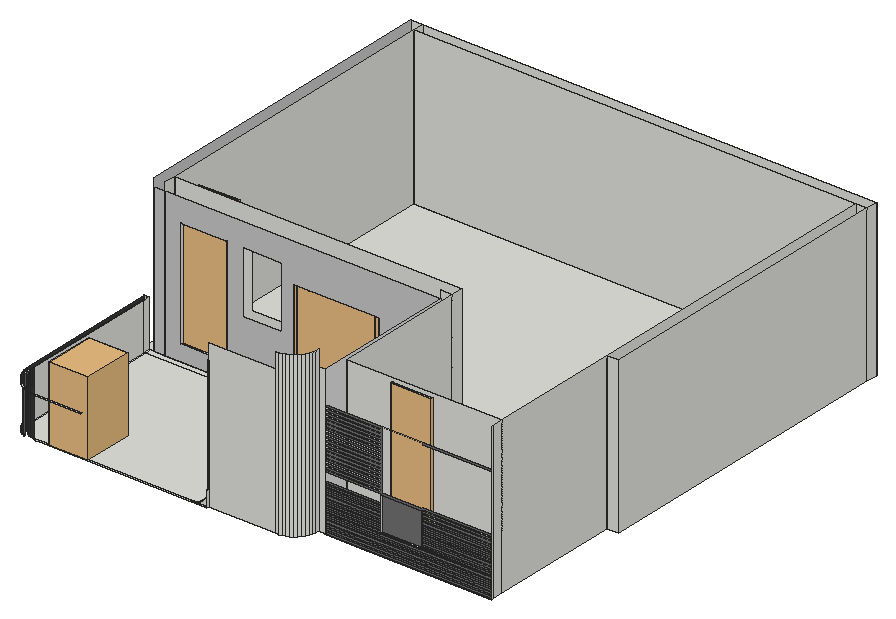
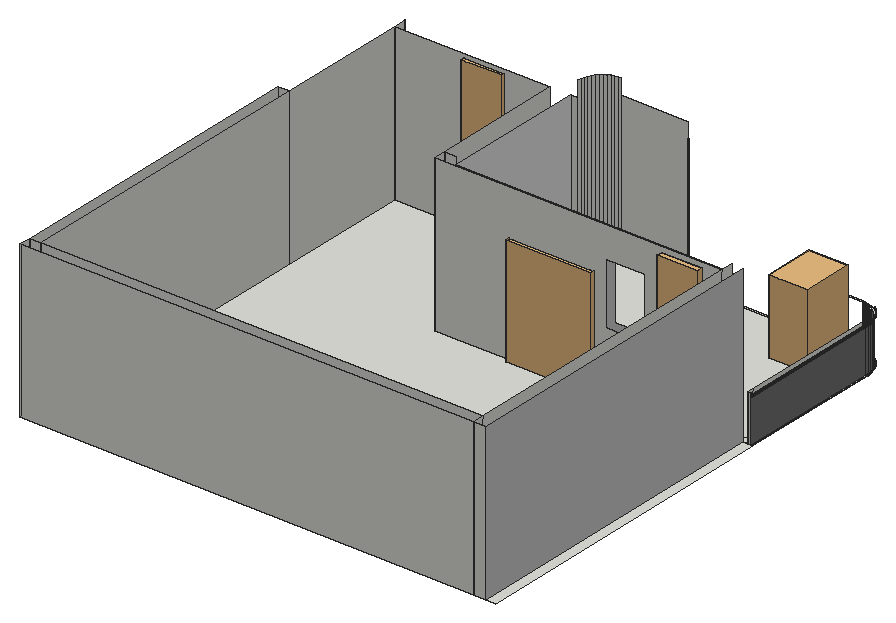
# SketchUp Ruby script. Lengths in inches.
U = 1.inch
M = Sketchup.active_model
def pt(a) = Geom::Point3d.new(a.map { |v| v * U })
def face(e, loops, mat)
  f = e.add_face(loops[0].map { |a| pt(a) })
  loops[1..].each { |l| e.add_face(l.map { |a| pt(a) }).erase! }
  f.material = f.back_material = mat if mat
  f
end
# faces: each face lists its corners as indices into pts; further lists are holes
def faces(e, pts, list, mat = nil) = list.each { |f| face(e, (f[0].is_a?(Array) ? f : [f]).map { |l| l.map { |i| pts[i] } }, mat) }
# xy, xz, yz: faces in a plane at the given z, y or x. An outline is a flat list of corners, or four numbers for a rectangle; further outlines are holes
def ring(l) = l.size == 4 ? [[l[0], l[1]], [l[2], l[1]], [l[2], l[3]], [l[0], l[3]]] : l.each_slice(2).to_a
def flat(e, list, mat, &to3) = list.each { |f| face(e, (f[0].is_a?(Array) ? f : [f]).map { |l| ring(l).map { |u, v| to3.(u, v) } }, mat) }
def xy(e, z, list, mat = nil) = flat(e, list, mat) { |x, y| [x, y, z] }
def xz(e, y, list, mat = nil) = flat(e, list, mat) { |x, z| [x, y, z] }
def yz(e, x, list, mat = nil) = flat(e, list, mat) { |y, z| [x, y, z] }
def lines(e, pts, list) = list.each { |a, b| e.add_line(pt(pts[a]), pt(pts[b])) }
# prism: a flat outline (further loops are holes) pulled along v
def prism(e, loops, v, mat = nil)
  f = face(e, loops, mat); d = Geom::Vector3d.new(v.map { |x| x * U })
  f.pushpull(f.normal.samedirection?(d) ? d.length : -d.length)
end
def box(e, o, s, mat = nil) = prism(e, [[o, [o[0] + s[0], o[1], o[2]], [o[0] + s[0], o[1] + s[1], o[2]], [o[0], o[1] + s[1], o[2]]]], [0, 0, s[2]], mat)
def at(x, y, z, deg = 0) = Geom::Transformation.translation(pt([x, y, z])) * Geom::Transformation.rotation(ORIGIN, Z_AXIS, deg.degrees)
def axes(o, x, y, z) = Geom::Transformation.new([*x, 0, *y, 0, *z, 0, *pt(o).to_a, 1])
def part(name) = M.definitions.add(name)
# library, detail: a bought-in or finely detailed component or shape, given as its bounding box
def library(name, o, s) = part(name).tap { |d| box(d.entities, o, s) }
def detail(e, o, s) = box(e.add_group.entities, o, s)
def put(e, d, t, mat = nil) = e.add_instance(d, t).tap { |i| i.material = mat if mat }
def group(e, t, mat = nil) = e.add_group.tap { |g| g.transformation = t; g.material = mat if mat }.entities
root = M.entities
M.materials.add("[Cladding Stucco White]").color = [200, 200, 200]
M.materials.add("[Color M01]").color = [226, 226, 226]
M.materials.add("[Color M05]").color = [114, 114, 114]
M.materials.add("[Color M07]").color = [58, 58, 58]
c1 = library("Potted Plant 02",[-16.98,-19.78,0],[30.04,38.68,37.52])
c2 = library("Curtains 004",[-15.59,-2.26,0],[31.18,4.52,116.91])
c3 = library("glass door",[0,-2.95,0],[39.37,5.9,82.68])
c4 = library("Door 243 053",[-21.6,-2.79,-0.07],[43.2,5.58,82.64])
xy(root,126,[[24.25,5.061,142.019,5.061,142.019,6.391,24.25,6.391,21.821,6.55,19.434,7.025,17.129,7.808,14.946,8.884,12.922,10.237,11.092,11.842,9.487,13.672,8.134,15.696,7.058,17.879,6.275,20.184,5.8,22.571,5.641,25,5.641,136,4.311,136,4.311,25,4.481,22.397,4.99,19.839,5.829,17.37,6.982,15.03,8.431,12.862,10.151,10.901,12.112,9.181,14.28,7.732,16.62,6.579,19.089,5.74,21.647,5.231],[142.019,5.061,154.019,6.391],[24.25,6.391,205.875,6.391,208.304,6.55,210.691,7.025,212.996,7.808,215.179,8.884,217.203,10.237,219.033,11.842,220.638,13.672,221.991,15.696,223.067,17.879,223.85,20.184,224.325,22.571,224.484,25,224.484,130.609,173.484,130.609,173.484,139.609,124.266,139.609,124.266,130.609,5.641,130.609,5.641,25,5.8,22.571,6.275,20.184,7.058,17.879,8.134,15.696,9.487,13.672,11.092,11.842,12.922,10.237,14.946,8.884,17.129,7.808,19.434,7.025,21.821,6.55],[229.875,24,238.875,25],[238.875,24,358.875,25],
  [224.484,25,229.875,25,229.875,136,178.875,136,178.875,145,118.875,145,118.875,136,5.641,136,5.641,130.609,124.266,130.609,124.266,139.609,173.484,139.609,173.484,130.609,224.484,130.609],[229.875,25,238.875,136],[238.875,25,358.875,34],[238.875,34,358.875,34,358.875,376,16.875,376,16.875,145,238.875,145],[0.25,136,7.875,385],
  [7.875,136,16.875,385],[16.875,136,118.875,145],[178.875,136,238.875,145],[358.875,136,367.875,376],[16.875,376,367.875,385]])
xy(root,126.103,[[12.811,5.186,12.812,5.189,10.324,6.851,10.322,6.849],[9.765,6.123,9.767,6.126,7.428,8.178,7.426,8.176],[10.322,6.849,10.324,6.851,8.074,8.824,8.072,8.822],[7.426,8.176,7.428,8.178,5.376,10.517,5.373,10.515],[8.072,8.822,8.074,8.824,6.101,11.074,6.099,11.072],
  [5.373,10.515,5.376,10.517,3.647,13.105,3.644,13.103],[6.099,11.072,6.101,11.074,4.439,13.562,4.436,13.561],[3.644,13.103,3.647,13.105,2.27,15.896,2.268,15.895],[4.436,13.561,4.439,13.562,3.115,16.246,3.113,16.245],[2.268,15.895,2.27,15.896,1.27,18.843,1.267,18.842],
  [3.113,16.245,3.115,16.246,2.153,19.079,2.151,19.078],[1.267,18.842,1.27,18.843,0.663,21.895,0.66,21.894],[2.151,19.078,2.153,19.079,1.57,22.014,1.567,22.014],[0.66,21.894,0.663,21.895,0.462,24.963,0.459,24.963],[0.459,24.963,0.462,24.963,0.459,25.007]])
xy(root,126.14,[[12.755,5.09,12.756,5.093,10.256,6.763,10.255,6.761],[9.833,6.211,9.835,6.214,7.506,8.256,7.504,8.254],[10.255,6.761,10.256,6.763,7.996,8.746,7.994,8.744],[7.504,8.254,7.506,8.256,5.464,10.585,5.461,10.583],[7.994,8.744,7.996,8.746,6.013,11.006,6.011,11.005],
  [5.461,10.583,5.464,10.585,3.743,13.16,3.74,13.159],[6.011,11.005,6.013,11.006,4.343,13.506,4.34,13.505],[3.74,13.159,3.743,13.16,2.373,15.938,2.37,15.937],[4.34,13.505,4.343,13.506,3.013,16.203,3.01,16.202],[2.37,15.937,2.373,15.938,1.377,18.871,1.374,18.871],
  [3.01,16.202,3.013,16.203,2.046,19.051,2.043,19.05],[1.374,18.871,1.377,18.871,0.773,21.909,0.77,21.909],[2.043,19.05,2.046,19.051,1.46,22,1.457,21.999],[0.77,21.909,0.773,21.909,0.572,24.967,0.57,24.967],[0.57,24.967,0.572,24.967,0.57,25.01]])
xy(root,126.166,[[12.698,4.992,12.7,4.994,10.187,6.673,10.185,6.671],[9.902,6.302,9.904,6.304,7.586,8.336,7.584,8.334],[10.185,6.671,10.187,6.673,7.915,8.665,7.913,8.663],[7.584,8.334,7.586,8.336,5.554,10.654,5.552,10.652],[7.913,8.663,7.915,8.665,5.923,10.937,5.921,10.935],
  [5.552,10.652,5.554,10.654,3.841,13.217,3.839,13.216],[5.921,10.935,5.923,10.937,4.244,13.45,4.242,13.448],[3.839,13.216,3.841,13.217,2.478,15.982,2.475,15.981],[4.242,13.448,4.244,13.45,2.908,16.16,2.905,16.159],[2.475,15.981,2.478,15.982,1.487,18.901,1.484,18.9],
  [2.905,16.159,2.908,16.16,1.936,19.021,1.934,19.02],[1.484,18.9,1.487,18.901,0.886,21.924,0.883,21.924],[1.934,19.02,1.936,19.021,1.347,21.985,1.344,21.984],[0.883,21.924,0.886,21.924,0.686,24.971,0.683,24.971],[1.344,21.984,1.347,21.985,1.15,24.986,1.147,24.986],
  [0.683,24.971,0.686,24.971,0.683,25.014],[1.147,24.986,1.15,24.986,1.147,25.029]])
xy(root,126.182,[[12.64,4.891,12.642,4.894,10.117,6.581,10.115,6.579],[9.973,6.394,9.974,6.396,7.668,8.418,7.666,8.416],[10.115,6.579,10.117,6.581,7.833,8.583,7.831,8.581],[7.666,8.416,7.668,8.418,5.646,10.724,5.644,10.723],[7.831,8.581,7.833,8.583,5.831,10.867,5.829,10.865],
  [5.644,10.723,5.646,10.724,3.942,13.275,3.939,13.274],[5.829,10.865,5.831,10.867,4.144,13.392,4.141,13.39],[3.939,13.274,3.942,13.275,2.585,16.026,2.582,16.025],[4.141,13.39,4.144,13.392,2.801,16.115,2.798,16.114],[2.582,16.025,2.585,16.026,1.599,18.931,1.596,18.93],
  [2.798,16.114,2.801,16.115,1.824,18.991,1.822,18.99],[1.596,18.93,1.599,18.931,1.001,21.939,0.998,21.939],[1.822,18.99,1.824,18.991,1.232,21.97,1.229,21.969],[0.998,21.939,1.001,21.939,0.802,24.975,0.799,24.974],[1.229,21.969,1.232,21.97,1.035,24.982,1.032,24.982],
  [0.799,24.974,0.802,24.975,0.799,25.018],[1.032,24.982,1.035,24.982,1.032,25.026]])
xy(root,126.1875,[[10.044,6.486,10.046,6.488,7.751,8.501,7.749,8.499],[7.749,8.499,7.751,8.501,5.738,10.796,5.736,10.794],[5.736,10.794,5.738,10.796,4.043,13.333,4.041,13.333,4.04,13.332],[4.04,13.332,4.041,13.333,4.043,13.333,2.693,16.071,2.691,16.07,2.69,16.07],[2.69,16.07,2.691,16.07,2.693,16.071,1.712,18.961,1.71,18.961,1.709,18.96],
  [1.709,18.96,1.71,18.961,1.712,18.961,1.116,21.954,1.113,21.954],[1.113,21.954,1.116,21.954,0.918,24.978,0.915,24.978],[0.915,24.978,0.918,24.978,0.915,25.022]])
xy(root,138,[[28.875,136,64.875,145]])
xy(root,141.966,[[272.513,25,304.568,26]])
xy(root,159.6875,[[24.217,1.33,21.16,1.531,18.123,2.135,15.191,3.13,12.414,4.5,9.84,6.22,7.512,8.262,5.47,10.59,3.75,13.164,2.38,15.941,1.385,18.873,0.781,21.91,0.58,24.967,0.58,135.75,1.58,135.75,1.58,25,1.774,22.041,2.353,19.133,3.306,16.325,4.618,13.665,6.265,11.2,8.22,8.97,10.45,7.015,12.915,5.368,15.575,4.056,18.383,3.103,21.291,2.524,24.25,2.33,59.529,2.33,59.529,1.33],[0.58,135.75,1.58,136]])
xz(root,6.391,[[142.019,126,143.585,126.103,145.124,126.409,146.611,126.913,148.019,127.608,149.324,128.48,150.504,129.515,151.539,130.695,152.411,132,153.105,133.408,153.61,134.894,153.916,136.434,154.019,138,154.019,126],[154.019,126,205.875,240]])
xz(root,25,[[224.484,126,229.875,240],[272.513,150.061,272.563,151.134],[272.513,152.561,272.563,153.634],[272.513,155.061,272.563,156.134],[272.513,157.561,272.563,158.634],
  [272.513,160.061,272.563,161.134]])
xz(root,25,[[229.875,126,358.875,127.561],[229.875,127.561,358.875,128.634],[229.875,128.634,358.875,130.123],[229.875,130.123,358.875,131.196],[229.875,131.196,358.875,132.686],
  [229.875,132.686,358.875,133.759],[229.875,133.759,358.875,135.248],[229.875,135.248,358.875,136.321],[229.875,136.321,358.875,137.811],[229.875,137.811,358.875,138.884],
  [229.875,138.884,358.875,140.373],[229.875,140.373,358.875,141.446],[229.875,141.446,358.875,141.446,358.875,142.311,304.619,142.311,304.619,143.384,358.875,143.384,358.875,144.83,304.619,144.83,304.619,145.904,358.875,145.904,358.875,147.561,304.619,147.561,304.619,148.634,358.875,148.634,358.875,150.123,304.619,150.123,304.619,151.196,358.875,151.196,358.875,152.248,304.619,152.248,304.619,153.321,358.875,153.321,358.875,154.873,304.619,154.873,304.619,155.946,358.875,155.946,358.875,157.498,304.619,157.498,304.619,158.571,358.875,158.571,358.875,160.123,304.619,160.123,304.619,161.196,358.875,161.196,358.875,162.748,304.619,162.748,304.619,163.821,358.875,163.821,358.875,165.373,304.619,165.373,304.619,166.446,358.875,166.446,358.875,167.873,304.619,167.873,304.619,168.946,358.875,168.946,358.875,170.373,304.626,170.373,304.626,169.2,273.063,169.2,273.063,215.012,304.626,215.012,304.626,213.946,358.875,213.946,358.875,215.373,229.875,215.373,229.875,213.759,272.563,213.759,272.563,212.686,229.875,212.686,229.875,211.071,272.563,211.071,272.563,209.998,229.875,209.998,229.875,208.384,272.563,208.384,272.563,207.311,229.875,207.311,229.875,205.696,272.563,205.696,272.563,204.623,229.875,204.623,229.875,203.009,272.563,203.009,272.563,201.936,229.875,201.936,229.875,200.321,272.563,200.321,272.563,199.248,229.875,199.248,229.875,197.634,272.563,197.634,272.563,196.561,229.875,196.561,229.875,194.946,272.563,194.946,272.563,193.873,229.875,193.873,229.875,192.259,272.563,192.259,272.563,191.186,229.875,191.186,229.875,189.571,272.563,189.571,272.563,188.498,229.875,188.498,229.875,186.884,272.563,186.884,272.563,185.811,229.875,185.811,229.875,184.196,272.563,184.196,272.563,183.123,229.875,183.123,229.875,181.509,272.563,181.509,272.563,180.436,229.875,180.436,229.875,178.821,272.563,178.821,272.563,177.748,229.875,177.748,229.875,176.134,272.563,176.134,272.563,175.061,229.875,175.061,229.875,173.634,272.563,173.634,272.563,172.561,229.875,172.561,229.875,171.134,272.563,171.134,272.563,170.061,229.875,170.061,229.875,168.634,272.563,168.634,272.563,167.904,304.568,167.904,304.568,141.966,272.513,141.966,272.513,142.748,229.875,142.748],[304.619,142.311,358.875,143.384],[229.875,142.748,272.513,143.821],
  [229.875,143.821,272.513,145.061],[304.619,144.83,358.875,145.904],[229.875,145.061,272.513,146.134],[229.875,146.134,272.513,147.498],[229.875,147.498,272.513,148.571],
  [304.619,147.561,358.875,148.634],[229.875,148.571,272.513,150.061],[229.875,150.061,272.513,151.134],[304.619,150.123,358.875,151.196],[229.875,151.134,272.513,152.561],
  [304.619,152.248,358.875,153.321],[229.875,152.561,272.513,153.634],[229.875,153.634,272.513,155.061],[304.619,154.873,358.875,155.946],[229.875,155.061,272.513,156.134],
  [229.875,156.134,272.513,157.561],[304.619,157.498,358.875,158.571],[229.875,157.561,272.513,158.634],[229.875,158.634,272.513,160.061],[229.875,160.061,272.513,161.134],
  [304.619,160.123,358.875,161.196],[229.875,161.134,272.513,162.561]],"[Color M05]")
xz(root,26,[[272.513,141.966,304.568,167.904]],"[Color M05]")
xz(root,34,[[[238.875,126,358.875,246],[273.063,169.2,304.626,215.012]]])
xz(root,135.75,[[0.58,159.6875,1.58,162]])
xz(root,136,[[1.58,126,4.311,162],[229.875,126,238.875,246],[358.875,126,367.875,246],[0.58,159.6875,1.58,162]])
xz(root,136,[[7.875,126,16.875,240],[[16.875,126,118.875,126,118.875,210,178.875,210,178.875,126,229.875,126,229.875,240,16.875,240],[28.875,138,64.875,222],[76.875,174,106.875,222]]],"[Cladding Stucco White]")
xz(root,145,[[[16.875,126,16.875,246,238.875,246,238.875,126,178.875,126,178.875,210,118.875,210,118.875,126],[28.875,138,64.875,222],[76.875,174,106.875,222]]])
xz(root,376,[[16.875,126,358.875,246],[358.875,126,367.875,246]])
xz(root,385,[[7.875,126,16.875,246],[16.875,126,367.875,246]])
yz(root,0.58,[[135.75,159.6875,136,162]])
yz(root,0.58,[[24.967,159.6875,135.75,162]],"[Color M07]")
yz(root,1.58,[[135.75,159.6875,136,162]])
yz(root,1.58,[[25,126,136,159.6875]],"[Color M05]")
yz(root,4.311,[[25,126,130.609,162],[130.609,126,136,162]])
yz(root,7.875,[[136,126,385,246]],"[Cladding Stucco White]")
yz(root,16.875,[[136,126,145,246],[145,126,376,246],[376,126,385,246]])
yz(root,28.875,[[136,138,145,222]])
yz(root,64.875,[[136,138,145,222]])
yz(root,118.875,[[136,126,145,210]])
yz(root,154.019,[[5.061,126,6.391,138]])
yz(root,178.875,[[136,126,145,210]])
yz(root,229.875,[[25,126,136,240]],"[Color M01]")
yz(root,238.875,[[34,126,136,246],[136,126,145,246]])
yz(root,272.513,[[25,141.966,26,167.904]])
yz(root,304.568,[[25,141.966,26,167.904]])
yz(root,358.875,[[24,126,25,246],[25,126,34,246],[34,126,136,246],[136,126,376,246]])
yz(root,367.875,[[136,126,376,246],[376,126,385,246]])
p = [[10.45,7.015,126],[10.387,6.934,126.056],[12.864,5.279,126.056],[12.915,5.368,126],[12.915,5.368,126.002],[12.917,5.37,126],
  [10.451,7.017,126],[10.45,7.015,126.002],[10.389,6.936,126.056],[12.865,5.281,126.056],[12.915,5.368,159.6875],[10.45,7.015,159.6875],
  [19.089,5.74,126],[16.62,6.579,126],[16.62,6.579,162],[19.089,5.74,162],[7.35,8.1,126.056],[7.277,8.027,126],
  [9.638,5.957,126],[9.7,6.038,126.056],[9.64,5.96,126],[9.702,6.041,126.056],[7.352,8.102,126.056],[7.279,8.029,126],
  [143.576,6.175,126.171],[143.58,6.284,126.14],[142.123,6.284,126.045],[142.23,6.175,126.083],[143.585,6.391,126.103],[142.019,6.391,126],
  [208.304,6.55,126],[205.875,6.391,126],[205.875,6.391,240],[205.875,6.391,252],[208.304,6.55,252],[14.28,7.732,126],
  [14.28,7.732,162],[210.691,7.025,126],[210.691,7.025,252],[8.22,8.97,126],[8.148,8.898,126.056],[8.222,8.972,126],
  [8.22,8.97,126.002],[8.15,8.9,126.056],[8.22,8.97,159.6875],[212.996,7.808,126],[212.996,7.808,252],[12.112,9.181,126],
  [12.112,9.181,162],[215.179,8.884,126],[215.179,8.884,252],[5.288,10.45,126.056],[5.207,10.388,126],[5.291,10.452,126.056],
  [5.21,10.39,126],[6.265,11.2,126],[6.184,11.137,126.056],[6.267,11.201,126],[6.265,11.2,126.002],[6.186,11.139,126.056],
  [217.203,10.237,126],[217.203,10.237,252],[6.265,11.2,159.6875],[10.151,10.901,126],[10.151,10.901,162],[219.033,11.842,126],
  [219.033,11.842,252],[3.552,13.05,126.056],[3.463,12.999,126],[3.554,13.051,126.056],[3.465,13,126],[8.431,12.862,126],
  [8.431,12.862,162],[4.618,13.665,126],[4.529,13.614,126.056],[4.62,13.667,126],[4.618,13.665,126.002],[4.531,13.615,126.056],
  [4.618,13.665,159.6875],[220.638,13.672,126],[220.638,13.672,252],[6.982,15.03,126],[6.982,15.03,162],[2.169,15.854,126.056],
  [2.074,15.815,126],[2.171,15.855,126.056],[2.077,15.816,126],[3.306,16.325,126],[3.211,16.286,126.056],[3.309,16.326,126],
  [3.306,16.325,126.002],[3.214,16.287,126.056],[3.306,16.325,159.6875],[221.991,15.696,126],[221.991,15.696,252],[5.829,17.37,126],
  [5.829,17.37,162],[223.067,17.879,126],[223.067,17.879,252],[1.164,18.814,126.056],[1.065,18.788,126],[1.167,18.815,126.056],
  [1.068,18.788,126],[2.353,19.133,126],[2.254,19.106,126.056],[2.356,19.133,126],[2.353,19.133,126.002],[2.257,19.107,126.056],
  [2.353,19.133,159.6875],[4.99,19.839,126],[4.99,19.839,162],[223.85,20.184,126],[223.85,20.184,252],[0.554,21.88,126.056],
  [0.452,21.867,126],[0.557,21.881,126.056],[0.455,21.867,126],[1.774,22.041,126],[1.673,22.028,126.056],[1.777,22.041,126],
  [1.774,22.041,126.002],[1.676,22.028,126.056],[1.774,22.041,159.6875],[4.481,22.397,126],[4.481,22.397,162],[224.325,22.571,126],
  [224.325,22.571,252],[0.352,24.96,126.056],[0.25,24.956,126],[0.352,25.003,126.056],[0.25,25,126],[1.58,25.044,126],
  [1.478,25.04,126.056],[1.58,25,126],[1.478,24.997,126.056],[1.58,25,159.6875],[4.311,25,126],[4.311,25,162],
  [224.484,25,126],[224.484,25,252],[224.484,25,240],[0.25,134.67,126],[0.352,134.772,126.056],[0.352,135.898,126.056],
  [0.25,136,126],[1.478,134.772,126.056],[1.58,134.67,126],[1.58,136,126],[1.478,135.898,126.056],[10.255,6.761,126.14],
  [10.187,6.673,126.166],[12.7,4.994,126.166],[12.755,5.09,126.14],[10.322,6.849,126.103],[10.256,6.763,126.14],[12.756,5.093,126.14],
  [12.811,5.186,126.103],[12.812,5.189,126.103],[10.324,6.851,126.103],[143.569,5.839,126.223],[143.57,5.952,126.213],[142.449,5.952,126.139],
  [142.561,5.839,126.157],[7.426,8.176,126.103],[9.765,6.123,126.103],[9.767,6.126,126.103],[7.428,8.178,126.103],[143.573,6.064,126.195],
  [142.339,6.064,126.114],[7.504,8.254,126.14],[9.833,6.211,126.14],[7.584,8.334,126.166],[7.506,8.256,126.14],[9.835,6.214,126.14],
  [9.902,6.302,126.166],[145.106,6.175,126.476],[145.115,6.284,126.445],[145.124,6.391,126.409],[7.994,8.744,126.14],[7.915,8.665,126.166],
  [8.072,8.822,126.103],[7.996,8.746,126.14],[8.074,8.824,126.103],[5.373,10.515,126.103],[5.376,10.517,126.103],[5.461,10.583,126.14],
  [5.552,10.652,126.166],[5.464,10.585,126.14],[6.011,11.005,126.14],[5.923,10.937,126.166],[6.099,11.072,126.103],[6.013,11.006,126.14],
  [6.101,11.074,126.103],[3.644,13.103,126.103],[3.647,13.105,126.103],[3.74,13.159,126.14],[3.839,13.216,126.166],[3.743,13.16,126.14],
  [4.34,13.505,126.14],[4.244,13.45,126.166],[4.436,13.561,126.103],[4.343,13.506,126.14],[4.439,13.562,126.103],[2.268,15.895,126.103],
  [2.27,15.896,126.103],[2.37,15.937,126.14],[2.475,15.981,126.166],[2.373,15.938,126.14],[3.01,16.202,126.14],[2.908,16.16,126.166],
  [3.113,16.245,126.103],[3.013,16.203,126.14],[3.115,16.246,126.103],[1.267,18.842,126.103],[1.27,18.843,126.103],[1.374,18.871,126.14],
  [1.484,18.9,126.166],[1.377,18.871,126.14],[2.043,19.05,126.14],[1.936,19.021,126.166],[2.151,19.078,126.103],[2.046,19.051,126.14],
  [2.153,19.079,126.103],[0.66,21.894,126.103],[0.663,21.895,126.103],[0.77,21.909,126.14],[0.883,21.924,126.166],[0.773,21.909,126.14],
  [1.457,21.999,126.14],[1.347,21.985,126.166],[1.567,22.014,126.103],[1.46,22,126.14],[1.57,22.014,126.103],[0.459,24.963,126.103],
  [0.462,24.963,126.103],[0.459,25.007,126.103],[0.57,24.967,126.14],[0.572,24.967,126.14],[0.57,25.01,126.14],[0.683,24.971,126.166],
  [0.886,21.924,126.166],[0.686,24.971,126.166],[0.683,25.014,126.166],[1.261,24.99,126.14],[1.15,24.986,126.166],[1.263,24.99,126.139],
  [1.261,25.033,126.14],[1.147,25.029,126.166],[1.371,24.993,126.103],[1.371,25.037,126.103],[0.459,134.879,126.103],[0.459,135.791,126.103],
  [0.57,134.989,126.14],[0.57,135.68,126.14],[0.683,135.103,126.166],[0.683,135.567,126.166],[1.147,135.103,126.166],[1.261,134.989,126.14],
  [1.261,135.68,126.14],[1.147,135.567,126.166],[1.371,134.879,126.103],[1.371,135.791,126.103],[10.115,6.579,126.182],[10.046,6.488,126.1875],
  [12.583,4.793,126.1875],[12.64,4.891,126.182],[10.185,6.671,126.166],[10.117,6.581,126.182],[12.642,4.894,126.182],[12.698,4.992,126.166],
  [143.569,5.726,126.227],[142.674,5.726,126.168],[145.092,5.726,126.53],[145.093,5.839,126.526],[145.096,5.952,126.516],[145.1,6.064,126.499],
  [7.666,8.416,126.182],[7.586,8.336,126.166],[9.904,6.304,126.166],[9.973,6.394,126.182],[7.749,8.499,126.1875],[7.668,8.418,126.182],
  [9.974,6.396,126.182],[10.044,6.486,126.1875],[7.831,8.581,126.182],[7.751,8.501,126.1875],[7.913,8.663,126.166],[7.833,8.583,126.182],
  [5.644,10.723,126.182],[5.554,10.654,126.166],[5.736,10.794,126.1875],[5.646,10.724,126.182],[5.829,10.865,126.182],[5.738,10.796,126.1875],
  [5.921,10.935,126.166],[5.831,10.867,126.182],[3.939,13.274,126.182],[3.841,13.217,126.166],[4.04,13.332,126.1875],[3.942,13.275,126.182],
  [4.141,13.39,126.182],[4.043,13.333,126.1875],[4.242,13.448,126.166],[4.144,13.392,126.182],[2.582,16.025,126.182],[2.478,15.982,126.166],
  [2.69,16.07,126.1875],[2.585,16.026,126.182],[2.798,16.114,126.182],[2.693,16.071,126.1875],[2.905,16.159,126.166],[2.801,16.115,126.182],
  [1.596,18.93,126.182],[1.487,18.901,126.166],[1.709,18.96,126.1875],[1.599,18.931,126.182],[1.822,18.99,126.182],[1.712,18.961,126.1875],
  [1.934,19.02,126.166],[1.824,18.991,126.182],[0.998,21.939,126.182],[1.113,21.954,126.1875],[1.001,21.939,126.182],[1.229,21.969,126.182],
  [1.116,21.954,126.1875],[1.344,21.984,126.166],[1.232,21.97,126.182],[0.799,24.974,126.182],[0.802,24.975,126.182],[0.799,25.018,126.182],
  [0.915,24.978,126.1875],[1.115,21.954,126.1875],[0.918,24.978,126.1875],[0.915,25.022,126.1875],[1.032,24.982,126.182],[1.035,24.982,126.182],
  [1.032,25.026,126.182],[1.147,24.986,126.166],[0.799,135.218,126.182],[0.799,135.451,126.182],[0.915,135.335,126.1875],[1.032,135.218,126.182],
  [1.032,135.451,126.182],[146.584,6.175,126.977],[146.596,6.284,126.948],[146.611,6.391,126.913],[146.563,5.726,127.029],[146.564,5.839,127.026],
  [146.568,5.952,127.016],[146.575,6.064,127],[147.984,6.175,127.668],[148,6.284,127.641],[148.019,6.391,127.608],[147.956,5.726,127.716],
  [147.958,5.839,127.713],[147.963,5.952,127.704],[147.972,6.064,127.689],[149.282,6.175,128.535],[149.301,6.284,128.51],[149.324,6.391,128.48],
  [149.248,5.726,128.579],[149.25,5.839,128.576],[149.256,5.952,128.568],[149.267,6.064,128.554],[150.438,6.064,129.581],[150.455,6.175,129.564],
  [150.477,6.284,129.542],[150.504,6.391,129.515],[150.415,5.726,129.603],[150.418,5.839,129.601],[150.425,5.952,129.593],[151.484,6.175,130.737],
  [151.509,6.284,130.718],[151.539,6.391,130.695],[151.442,5.613,130.769],[151.44,5.726,130.771],[150.418,5.613,129.601],[151.442,5.839,130.769],
  [151.451,5.952,130.762],[151.465,6.064,130.752],[152.33,6.064,132.047],[152.351,6.175,132.035],[152.378,6.284,132.019],[152.411,6.391,132],
  [152.306,5.613,132.061],[152.303,5.726,132.0625],[152.306,5.839,132.061],[152.315,5.952,132.055],[153.003,5.952,133.45],[153.019,6.064,133.444],
  [153.041,6.175,133.434],[153.07,6.284,133.422],[153.105,6.391,133.408],[152.993,5.613,133.454],[152.99,5.726,133.456],[152.993,5.839,133.454],
  [153.502,5.952,134.923],[153.519,6.064,134.918],[153.543,6.175,134.912],[153.573,6.284,134.904],[153.61,6.391,134.894],[153.492,5.613,134.926],
  [153.489,5.726,134.927],[153.492,5.839,134.926],[153.795,5.613,136.45],[153.792,5.726,136.45],[153.795,5.839,136.45],[153.806,5.952,136.448],
  [153.823,6.064,136.446],[153.847,6.175,136.443],[153.878,6.284,136.439],[153.916,6.391,136.434],[153.847,5.613,137.231],[153.851,5.726,137.344],
  [153.861,5.839,137.457],[153.879,5.952,137.569],[153.904,6.064,137.68],[153.936,6.175,137.789],[153.974,6.284,137.896],[154.019,6.391,138],
  [154.001,6.281,138.11],[154.019,5.061,138],[154.001,5.171,138.11],[154.001,6.281,227.89],[154.019,6.391,228],[154.019,6.391,163.33],
  [154.019,6.391,139.33],[154.001,6.281,139.221],[154.001,6.281,163.221],[153.987,6.171,138.22],[153.987,5.281,138.22],[153.987,6.171,227.78],
  [153.987,6.171,139.11],[153.987,6.171,163.11],[153.975,6.06,138.331],[153.975,5.392,138.331],[153.975,6.06,138.999],[153.975,6.06,162.999],
  [153.975,6.06,227.669],[153.967,5.949,138.442],[153.967,5.503,138.442],[153.967,5.949,138.888],[153.967,5.949,162.888],[153.967,5.949,227.558],
  [153.963,5.838,138.554],[153.963,5.615,138.554],[153.963,5.838,138.777],[153.963,5.838,162.777],[153.963,5.838,227.446],[153.961,5.726,138.665],
  [153.961,5.726,227.335],[153.961,5.726,162.665],[7.512,8.262,162],[7.512,8.262,159.6875],[9.84,6.22,159.6875],[9.84,6.22,162],
  [5.47,10.59,162],[5.47,10.59,159.6875],[3.75,13.164,162],[3.75,13.164,159.6875],[2.38,15.941,162],[2.38,15.941,159.6875],
  [1.385,18.873,162],[1.385,18.873,159.6875],[0.781,21.91,162],[0.781,21.91,159.6875],[0.58,24.967,162],[0.58,24.967,159.6875]]
faces(root,p,[[0,1,2,3],[4,5,6,7,8,9],[16,17,18,19],[20,21,22,23],[24,25,26,27],[25,28,29,26],[30,31,32,33,34],[37,30,34,38],
  [39,40,1,0],[7,6,41,42,43,8],[45,37,38,46],[49,45,46,50],[51,52,17,16],[23,22,53,54],[55,56,40,39],[42,41,57,58,59,43],
  [60,49,50,61],[65,60,61,66],[67,68,52,51],[54,53,69,70],[73,74,56,55],[58,57,75,76,77,59],[79,65,66,80],[83,84,68,67],
  [70,69,85,86],[87,88,74,73],[76,75,89,90,91,77],[93,79,80,94],[97,93,94,98],[99,100,84,83],[86,85,101,102],[103,104,88,87],
  [90,89,105,106,107,91],[111,97,98,112],[113,114,100,99],[102,101,115,116],[117,118,104,103],[106,105,119,120,121,107],[125,111,112,126],[127,128,114,113],
  [116,115,129,130],[120,119,131,132,121],[133,134,118,117],[138,125,126,139,140],[141,130,128,127,129,142,143,144],[133,131,132,134],[145,132,131,146,147,148],[144,143,148,147],
  [149,150,151,152],[153,154,155,156],[1,153,156,2],[157,9,8,158],[159,160,161,162],[163,16,19,164],[21,165,166,22],[160,167,168,161],
  [169,166,165,170],[167,24,27,168],[171,172,173,174],[175,176,25,24],[176,177,28,25],[178,179,150,149],[180,181,154,153],[40,180,153,1],
  [158,8,43,182],[183,51,16,163],[22,166,184,53],[185,184,166,169],[186,187,172,171],[188,189,179,178],[190,191,181,180],[56,190,180,40],
  [182,43,59,192],[193,67,51,183],[53,184,194,69],[195,194,184,185],[196,197,187,186],[198,199,189,188],[200,201,191,190],[74,200,190,56],
  [192,59,77,202],[203,83,67,193],[69,194,204,85],[205,204,194,195],[206,207,197,196],[199,198,208,209],[201,200,210,211],[88,210,200,74],
  [202,77,91,212],[213,99,83,203],[85,204,214,101],[204,205,215,214],[207,206,216,217],[209,208,218,219],[211,210,220,221],[104,220,210,88],
  [212,91,107,222],[223,113,99,213],[101,214,224,115],[214,215,225,224],[217,216,226,227],[219,218,228,229],[221,220,230,231],[118,230,220,104],
  [222,107,121,232],[233,127,113,223],[115,224,234,235,129],[236,234,224,225],[225,227,237,238,235,234,224],[239,237,227,226],[226,240,241,242,238,237,227],[243,244,229,228],
  [228,231,245,246,247,244,229],[228,231,245,243],[248,245,231,230],[230,232,249,246,245,231],[134,248,230,118],[232,121,132,249],[142,129,127,233,235,250,251,143],[250,235,234,236,238,252,253,251],
  [252,238,237,239,242,254,255,253],[256,247,244,243,246,257,258,259],[243,245,246],[257,246,245,248,249,260,261,258],[148,261,260,249,248,134,132,145],[253,255,259,258],[251,253,258,261],[143,251,261,148],
  [262,263,264,265],[266,267,268,269],[270,159,162,271],[272,273,159,270],[273,274,160,159],[274,275,167,160],[275,175,24,167],[276,277,278,279],
  [280,281,282,283],[284,285,263,262],[286,287,267,266],[288,289,277,276],[290,291,281,280],[292,293,285,284],[294,295,287,286],[296,297,289,288],
  [298,299,291,290],[300,301,293,292],[302,303,295,294],[304,305,297,296],[306,307,299,298],[308,309,301,300],[303,302,310,311],[305,304,312,313],
  [307,306,314,315],[309,308,316,317],[311,310,318,319],[313,312,320,240],[315,314,321,322],[317,316,323,324],[319,318,325,326],[327,241,240,320],
  [320,322,328,329,242,241,240],[330,328,322,321],[331,324,332,333,329,328,322,321],[334,332,324,323],[323,326,335,336,333,332,324],[337,335,326,325],[325,229,244,247,336,335,326],[254,242,241,327,329,338,339,255],
  [338,329,328,330,333,340,339],[340,333,332,334,336,341,342],[341,336,335,337,247,256,259,342],[339,340,342],[255,339,342,259],[343,344,176,175],[344,345,177,176],[346,347,273,272],
  [347,348,274,273],[348,349,275,274],[349,343,175,275],[350,351,344,343],[351,352,345,344],[353,354,347,346],[354,355,348,347],[355,356,349,348],
  [356,350,343,349],[357,358,351,350],[358,359,352,351],[360,361,354,353],[361,362,355,354],[362,363,356,355],[363,357,350,356],[364,365,357,363],
  [365,366,358,357],[366,367,359,358],[368,369,361,360],[369,370,362,361],[370,364,363,362],[371,372,366,365],[372,373,367,366],[374,375,368,376],
  [375,377,369,368],[377,378,370,369],[378,379,364,370],[379,371,365,364],[380,381,371,379],[381,382,372,371],[382,383,373,372],[384,385,375,374],
  [385,386,377,375],[386,387,378,377],[387,380,379,378],[388,389,380,387],[389,390,381,380],[390,391,382,381],[391,392,383,382],[393,394,385,384],
  [394,395,386,385],[395,388,387,386],[396,397,389,388],[397,398,390,389],[398,399,391,390],[399,400,392,391],[401,402,394,393],[402,403,395,394],
  [403,396,388,395],[404,405,402,401],[405,406,403,402],[406,407,396,403],[407,408,397,396],[408,409,398,397],[409,410,399,398],[410,411,400,399],
  [412,413,405,404],[413,414,406,405],[414,415,407,406],[415,416,408,407],[416,417,409,408],[417,418,410,409],[418,419,411,410],[420,419,421,422],
  [423,424,425,426,419,420,427,428],[429,420,422,430],[431,423,428,427,420,429,432,433],[434,429,430,435],[436,437,438,431,433,432,429,434],[439,434,435,440],[441,442,443,438,437,436,434,439],[444,439,440,445],
  [446,447,448,443,442,441,439,444],[449,444,445],[450,448,447,446,444,449,451]])
faces(root,p,[[0,3,4,10,11,7],[39,0,7,11,44,42],[55,39,42,44,62,58],[73,55,58,62,78,76],[87,73,76,78,92,90],[103,87,90,92,108,106],[117,103,106,108,122,120],[133,117,120,122,135]],"[Color M05]")
faces(root,p,[[12,13,14,15],[13,35,36,14],[35,47,48,36],[47,63,64,48],[63,71,72,64],[71,81,82,72],[81,95,96,82],[95,109,110,96],
  [109,123,124,110],[123,136,137,124],[452,453,454,455],[456,457,453,452],[458,459,457,456],[460,461,459,458],[462,463,461,460],[464,465,463,462],
  [466,467,465,464]],"[Color M07]")
put(root,c1,axes([47.83,25.93,126],[1,0,0],[0,1,0],[0,0,1.53]))
put(root,c2,at(290.02,34.29,126))
put(root,c3,axes([28.875,139.93,138],[0.9144,0,0],[0,0.67,0],[0,0,1.016]))
put(root,c4,axes([149.15,141.89,126],[1.5125,0,0],[0,2.11547,0],[0,0,1.01736]))
put(root,c2,at(46.77,148.75,126))
